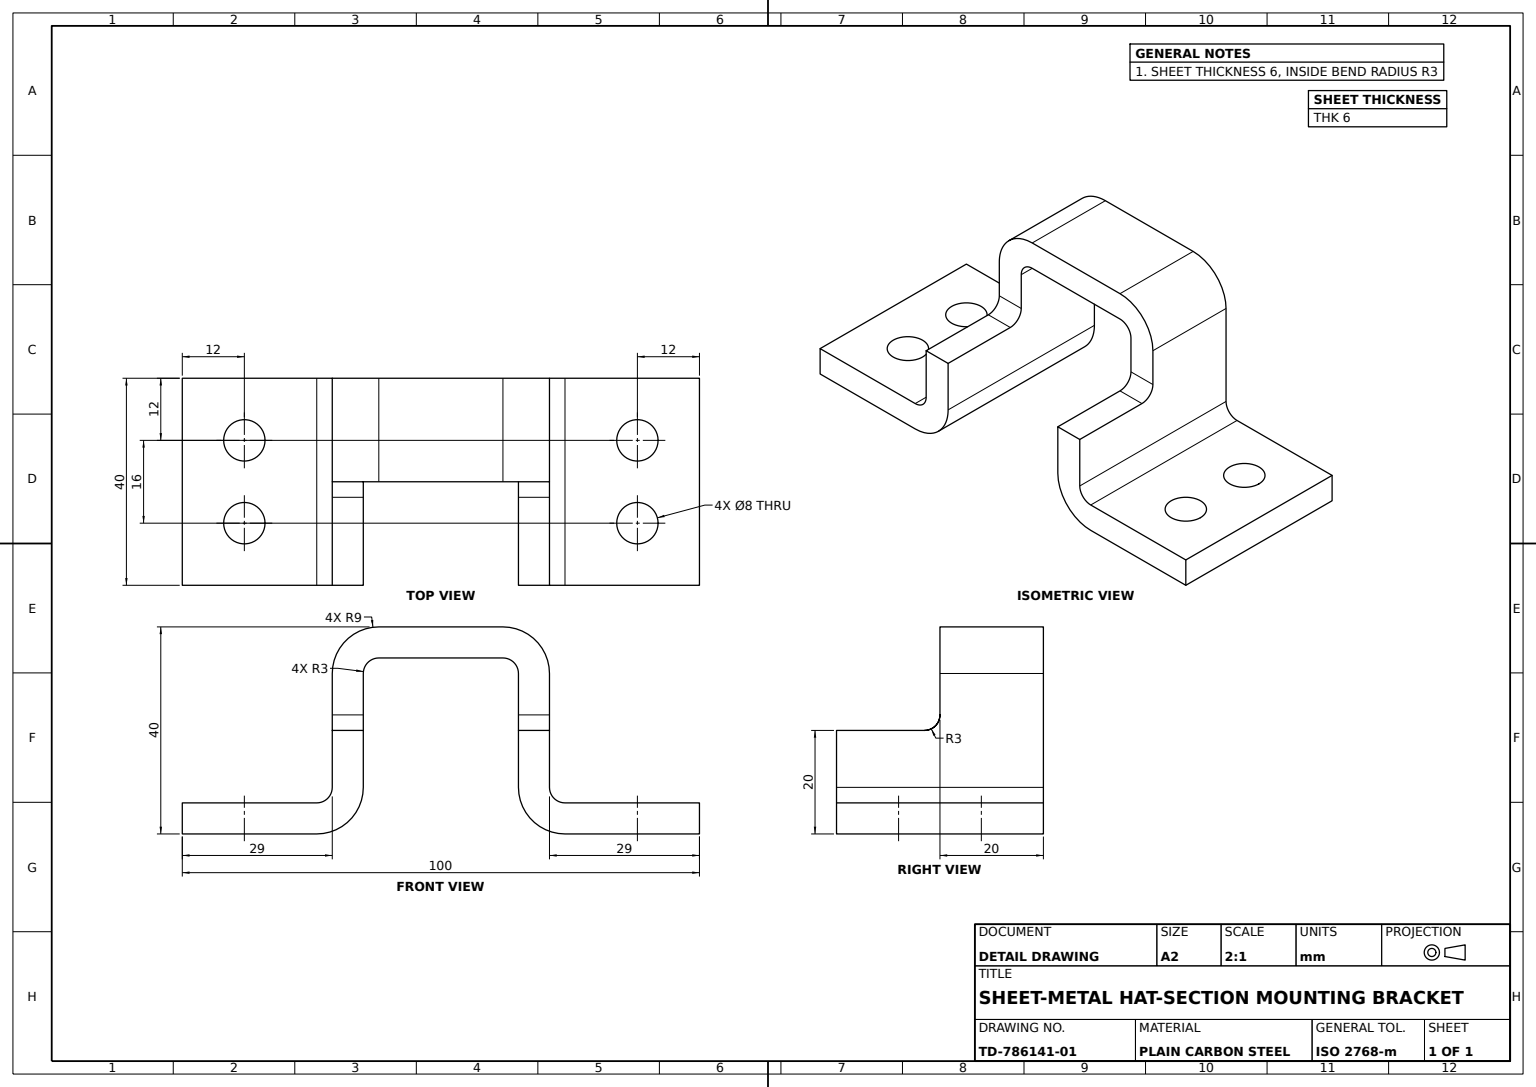
ISO-10303-21;
HEADER;
FILE_DESCRIPTION((''),'2;1');
FILE_NAME('','',(''),(''),'','','');
FILE_SCHEMA(('AUTOMOTIVE_DESIGN'));
ENDSEC;
DATA;
#1=APPLICATION_CONTEXT('');
#2=PRODUCT_CONTEXT('',#1,'mechanical');
#3=PRODUCT('','','',(#2));
#4=PRODUCT_DEFINITION_FORMATION('','',#3);
#5=PRODUCT_DEFINITION_CONTEXT('',#1,'design');
#6=PRODUCT_DEFINITION('','',#4,#5);
#7=PRODUCT_DEFINITION_SHAPE('','',#6);
#8=(LENGTH_UNIT()NAMED_UNIT(*)SI_UNIT(.MILLI.,.METRE.));
#9=(NAMED_UNIT(*)PLANE_ANGLE_UNIT()SI_UNIT($,.RADIAN.));
#10=(NAMED_UNIT(*)SI_UNIT($,.STERADIAN.)SOLID_ANGLE_UNIT());
#11=UNCERTAINTY_MEASURE_WITH_UNIT(LENGTH_MEASURE(1.E-05),#8,'distance_accuracy_value','');
#12=(GEOMETRIC_REPRESENTATION_CONTEXT(3)GLOBAL_UNCERTAINTY_ASSIGNED_CONTEXT((#11))GLOBAL_UNIT_ASSIGNED_CONTEXT((#8,#9,#10))REPRESENTATION_CONTEXT('',''));
#13=CARTESIAN_POINT('',(12.,6.,0.));
#14=VERTEX_POINT('',#13);
#15=CARTESIAN_POINT('',(12.,0.,0.));
#16=VERTEX_POINT('',#15);
#17=DIRECTION('',(0.,-1.,0.));
#18=VECTOR('',#17,1000.);
#19=LINE('',#13,#18);
#20=EDGE_CURVE('',#14,#16,#19,.T.);
#21=ORIENTED_EDGE('',*,*,#20,.F.);
#22=CARTESIAN_POINT('',(21.,-3.,0.));
#23=VERTEX_POINT('',#22);
#24=CARTESIAN_POINT('',(12.,-3.,0.));
#25=DIRECTION('',(0.,0.,-1.));
#26=DIRECTION('',(1.,0.,0.));
#27=AXIS2_PLACEMENT_3D('',#24,#25,#26);
#28=CIRCLE('',#27,9.);
#29=EDGE_CURVE('',#14,#23,#28,.T.);
#30=ORIENTED_EDGE('',*,*,#29,.T.);
#31=CARTESIAN_POINT('',(15.,-3.,0.));
#32=VERTEX_POINT('',#31);
#33=VECTOR('',#26,1000.);
#34=LINE('',#31,#33);
#35=EDGE_CURVE('',#32,#23,#34,.T.);
#36=ORIENTED_EDGE('',*,*,#35,.F.);
#37=CIRCLE('',#27,3.);
#38=EDGE_CURVE('',#16,#32,#37,.T.);
#39=ORIENTED_EDGE('',*,*,#38,.F.);
#40=EDGE_LOOP('',(#21,#30,#36,#39));
#41=FACE_OUTER_BOUND('',#40,.T.);
#42=DIRECTION('',(-1.,0.,0.));
#43=AXIS2_PLACEMENT_3D('',#31,#25,#42);
#44=PLANE('',#43);
#45=ADVANCED_FACE('',(#41),#44,.T.);
#46=CARTESIAN_POINT('',(-12.,6.,0.));
#47=VERTEX_POINT('',#46);
#48=CARTESIAN_POINT('',(15.,6.,0.));
#49=LINE('',#48,#33);
#50=EDGE_CURVE('',#47,#14,#49,.T.);
#51=ORIENTED_EDGE('',*,*,#50,.F.);
#52=CARTESIAN_POINT('',(-12.,6.,20.));
#53=VERTEX_POINT('',#52);
#54=CARTESIAN_POINT('',(-12.,6.,40.));
#55=VECTOR('',#25,1000.);
#56=LINE('',#54,#55);
#57=EDGE_CURVE('',#53,#47,#56,.T.);
#58=ORIENTED_EDGE('',*,*,#57,.F.);
#59=CARTESIAN_POINT('',(12.,6.,20.));
#60=VERTEX_POINT('',#59);
#61=CARTESIAN_POINT('',(-50.,6.,20.));
#62=LINE('',#61,#33);
#63=EDGE_CURVE('',#53,#60,#62,.T.);
#64=ORIENTED_EDGE('',*,*,#63,.T.);
#65=CARTESIAN_POINT('',(12.,6.,40.));
#66=LINE('',#65,#55);
#67=EDGE_CURVE('',#60,#14,#66,.T.);
#68=ORIENTED_EDGE('',*,*,#67,.T.);
#69=EDGE_LOOP('',(#51,#58,#64,#68));
#70=FACE_OUTER_BOUND('',#69,.T.);
#71=CARTESIAN_POINT('',(15.,6.,40.));
#72=DIRECTION('',(0.,1.,0.));
#73=DIRECTION('',(0.,0.,1.));
#74=AXIS2_PLACEMENT_3D('',#71,#72,#73);
#75=PLANE('',#74);
#76=ADVANCED_FACE('',(#70),#75,.T.);
#77=CARTESIAN_POINT('',(15.,-14.,40.));
#78=VERTEX_POINT('',#77);
#79=CARTESIAN_POINT('',(15.,-14.,23.));
#80=VERTEX_POINT('',#79);
#81=LINE('',#77,#55);
#82=EDGE_CURVE('',#78,#80,#81,.T.);
#83=ORIENTED_EDGE('',*,*,#82,.T.);
#84=CARTESIAN_POINT('',(15.,-11.,20.));
#85=VERTEX_POINT('',#84);
#86=CARTESIAN_POINT('',(15.,-11.,23.));
#87=AXIS2_PLACEMENT_3D('',#86,#26,#72);
#88=CIRCLE('',#87,3.);
#89=EDGE_CURVE('',#80,#85,#88,.T.);
#90=ORIENTED_EDGE('',*,*,#89,.T.);
#91=CARTESIAN_POINT('',(15.,-3.,20.));
#92=VERTEX_POINT('',#91);
#93=CARTESIAN_POINT('',(15.,0.,20.));
#94=VECTOR('',#72,1000.);
#95=LINE('',#93,#94);
#96=EDGE_CURVE('',#85,#92,#95,.T.);
#97=ORIENTED_EDGE('',*,*,#96,.T.);
#98=CARTESIAN_POINT('',(15.,-3.,40.));
#99=LINE('',#98,#55);
#100=EDGE_CURVE('',#92,#32,#99,.T.);
#101=ORIENTED_EDGE('',*,*,#100,.T.);
#102=CARTESIAN_POINT('',(15.,-25.,0.));
#103=VERTEX_POINT('',#102);
#104=CARTESIAN_POINT('',(15.,0.,0.));
#105=LINE('',#104,#18);
#106=EDGE_CURVE('',#32,#103,#105,.T.);
#107=ORIENTED_EDGE('',*,*,#106,.T.);
#108=CARTESIAN_POINT('',(15.,-25.,40.));
#109=VERTEX_POINT('',#108);
#110=LINE('',#108,#55);
#111=EDGE_CURVE('',#109,#103,#110,.T.);
#112=ORIENTED_EDGE('',*,*,#111,.F.);
#113=CARTESIAN_POINT('',(15.,0.,40.));
#114=LINE('',#113,#18);
#115=EDGE_CURVE('',#78,#109,#114,.T.);
#116=ORIENTED_EDGE('',*,*,#115,.F.);
#117=EDGE_LOOP('',(#83,#90,#97,#101,#107,#112,#116));
#118=FACE_OUTER_BOUND('',#117,.T.);
#119=AXIS2_PLACEMENT_3D('',#113,#26,#72);
#120=PLANE('',#119);
#121=ADVANCED_FACE('',(#118),#120,.F.);
#122=CARTESIAN_POINT('',(-50.,-34.,40.));
#123=VERTEX_POINT('',#122);
#124=CARTESIAN_POINT('',(-24.,-34.,40.));
#125=VERTEX_POINT('',#124);
#126=CARTESIAN_POINT('',(-15.,-34.,40.));
#127=LINE('',#126,#33);
#128=EDGE_CURVE('',#123,#125,#127,.T.);
#129=ORIENTED_EDGE('',*,*,#128,.T.);
#130=CARTESIAN_POINT('',(-24.,-28.,40.));
#131=VERTEX_POINT('',#130);
#132=LINE('',#124,#94);
#133=EDGE_CURVE('',#125,#131,#132,.T.);
#134=ORIENTED_EDGE('',*,*,#133,.T.);
#135=CARTESIAN_POINT('',(-50.,-28.,40.));
#136=VERTEX_POINT('',#135);
#137=CARTESIAN_POINT('',(-15.,-28.,40.));
#138=LINE('',#137,#33);
#139=EDGE_CURVE('',#136,#131,#138,.T.);
#140=ORIENTED_EDGE('',*,*,#139,.F.);
#141=LINE('',#122,#94);
#142=EDGE_CURVE('',#123,#136,#141,.T.);
#143=ORIENTED_EDGE('',*,*,#142,.F.);
#144=EDGE_LOOP('',(#129,#134,#140,#143));
#145=FACE_OUTER_BOUND('',#144,.T.);
#146=CARTESIAN_POINT('',(-21.,-25.,40.));
#147=AXIS2_PLACEMENT_3D('',#146,#73,#26);
#148=PLANE('',#147);
#149=ADVANCED_FACE('',(#145),#148,.T.);
#150=VERTEX_POINT('',#146);
#151=CARTESIAN_POINT('',(-24.,-25.,40.));
#152=AXIS2_PLACEMENT_3D('',#151,#73,#26);
#153=CIRCLE('',#152,3.);
#154=EDGE_CURVE('',#131,#150,#153,.T.);
#155=ORIENTED_EDGE('',*,*,#154,.T.);
#156=CARTESIAN_POINT('',(-21.,-25.,0.));
#157=VERTEX_POINT('',#156);
#158=LINE('',#146,#55);
#159=EDGE_CURVE('',#150,#157,#158,.T.);
#160=ORIENTED_EDGE('',*,*,#159,.T.);
#161=CARTESIAN_POINT('',(-24.,-28.,0.));
#162=VERTEX_POINT('',#161);
#163=CARTESIAN_POINT('',(-24.,-25.,0.));
#164=AXIS2_PLACEMENT_3D('',#163,#73,#26);
#165=CIRCLE('',#164,3.);
#166=EDGE_CURVE('',#162,#157,#165,.T.);
#167=ORIENTED_EDGE('',*,*,#166,.F.);
#168=LINE('',#130,#55);
#169=EDGE_CURVE('',#131,#162,#168,.T.);
#170=ORIENTED_EDGE('',*,*,#169,.F.);
#171=EDGE_LOOP('',(#155,#160,#167,#170));
#172=FACE_OUTER_BOUND('',#171,.T.);
#173=AXIS2_PLACEMENT_3D('',#151,#25,#42);
#174=CYLINDRICAL_SURFACE('',#173,3.);
#175=ADVANCED_FACE('',(#172),#174,.F.);
#176=CARTESIAN_POINT('',(-15.,-25.,40.));
#177=VERTEX_POINT('',#176);
#178=CARTESIAN_POINT('',(-15.,-25.,0.));
#179=VERTEX_POINT('',#178);
#180=LINE('',#176,#55);
#181=EDGE_CURVE('',#177,#179,#180,.T.);
#182=ORIENTED_EDGE('',*,*,#181,.F.);
#183=AXIS2_PLACEMENT_3D('',#151,#73,#42);
#184=CIRCLE('',#183,9.);
#185=EDGE_CURVE('',#125,#177,#184,.T.);
#186=ORIENTED_EDGE('',*,*,#185,.F.);
#187=CARTESIAN_POINT('',(-24.,-34.,0.));
#188=VERTEX_POINT('',#187);
#189=LINE('',#124,#55);
#190=EDGE_CURVE('',#125,#188,#189,.T.);
#191=ORIENTED_EDGE('',*,*,#190,.T.);
#192=AXIS2_PLACEMENT_3D('',#163,#73,#42);
#193=CIRCLE('',#192,9.);
#194=EDGE_CURVE('',#188,#179,#193,.T.);
#195=ORIENTED_EDGE('',*,*,#194,.T.);
#196=EDGE_LOOP('',(#182,#186,#191,#195));
#197=FACE_OUTER_BOUND('',#196,.T.);
#198=CYLINDRICAL_SURFACE('',#173,9.);
#199=ADVANCED_FACE('',(#197),#198,.T.);
#200=CARTESIAN_POINT('',(42.,-34.,12.));
#201=VERTEX_POINT('',#200);
#202=CARTESIAN_POINT('',(34.,-34.,12.));
#203=VERTEX_POINT('',#202);
#204=CARTESIAN_POINT('',(38.,-34.,12.));
#205=AXIS2_PLACEMENT_3D('',#204,#72,#42);
#206=CIRCLE('',#205,4.);
#207=EDGE_CURVE('',#201,#203,#206,.T.);
#208=ORIENTED_EDGE('',*,*,#207,.F.);
#209=CARTESIAN_POINT('',(42.,-28.,12.));
#210=VERTEX_POINT('',#209);
#211=LINE('',#200,#94);
#212=EDGE_CURVE('',#201,#210,#211,.T.);
#213=ORIENTED_EDGE('',*,*,#212,.T.);
#214=CARTESIAN_POINT('',(34.,-28.,12.));
#215=VERTEX_POINT('',#214);
#216=CARTESIAN_POINT('',(38.,-28.,12.));
#217=AXIS2_PLACEMENT_3D('',#216,#72,#42);
#218=CIRCLE('',#217,4.);
#219=EDGE_CURVE('',#210,#215,#218,.T.);
#220=ORIENTED_EDGE('',*,*,#219,.T.);
#221=LINE('',#202,#94);
#222=EDGE_CURVE('',#203,#215,#221,.T.);
#223=ORIENTED_EDGE('',*,*,#222,.F.);
#224=EDGE_LOOP('',(#208,#213,#220,#223));
#225=FACE_OUTER_BOUND('',#224,.T.);
#226=CYLINDRICAL_SURFACE('',#205,4.);
#227=ADVANCED_FACE('',(#225),#226,.F.);
#228=CARTESIAN_POINT('',(24.,-28.,40.));
#229=VERTEX_POINT('',#228);
#230=CARTESIAN_POINT('',(24.,-28.,0.));
#231=VERTEX_POINT('',#230);
#232=LINE('',#228,#55);
#233=EDGE_CURVE('',#229,#231,#232,.T.);
#234=ORIENTED_EDGE('',*,*,#233,.T.);
#235=CARTESIAN_POINT('',(21.,-25.,0.));
#236=VERTEX_POINT('',#235);
#237=CARTESIAN_POINT('',(24.,-25.,0.));
#238=AXIS2_PLACEMENT_3D('',#237,#73,#26);
#239=CIRCLE('',#238,3.);
#240=EDGE_CURVE('',#236,#231,#239,.T.);
#241=ORIENTED_EDGE('',*,*,#240,.F.);
#242=CARTESIAN_POINT('',(21.,-25.,40.));
#243=VERTEX_POINT('',#242);
#244=LINE('',#242,#55);
#245=EDGE_CURVE('',#243,#236,#244,.T.);
#246=ORIENTED_EDGE('',*,*,#245,.F.);
#247=CARTESIAN_POINT('',(24.,-25.,40.));
#248=AXIS2_PLACEMENT_3D('',#247,#73,#26);
#249=CIRCLE('',#248,3.);
#250=EDGE_CURVE('',#243,#229,#249,.T.);
#251=ORIENTED_EDGE('',*,*,#250,.T.);
#252=EDGE_LOOP('',(#234,#241,#246,#251));
#253=FACE_OUTER_BOUND('',#252,.T.);
#254=AXIS2_PLACEMENT_3D('',#247,#25,#42);
#255=CYLINDRICAL_SURFACE('',#254,3.);
#256=ADVANCED_FACE('',(#253),#255,.F.);
#257=CARTESIAN_POINT('',(-12.,0.,0.));
#258=VERTEX_POINT('',#257);
#259=LINE('',#257,#94);
#260=EDGE_CURVE('',#258,#47,#259,.T.);
#261=ORIENTED_EDGE('',*,*,#260,.T.);
#262=ORIENTED_EDGE('',*,*,#50,.T.);
#263=ORIENTED_EDGE('',*,*,#20,.T.);
#264=LINE('',#104,#33);
#265=EDGE_CURVE('',#258,#16,#264,.T.);
#266=ORIENTED_EDGE('',*,*,#265,.F.);
#267=EDGE_LOOP('',(#261,#262,#263,#266));
#268=FACE_OUTER_BOUND('',#267,.T.);
#269=CARTESIAN_POINT('',(-21.,-3.,0.));
#270=AXIS2_PLACEMENT_3D('',#269,#25,#42);
#271=PLANE('',#270);
#272=ADVANCED_FACE('',(#268),#271,.T.);
#273=LINE('',#161,#18);
#274=EDGE_CURVE('',#162,#188,#273,.T.);
#275=ORIENTED_EDGE('',*,*,#274,.T.);
#276=CARTESIAN_POINT('',(-50.,-34.,0.));
#277=VERTEX_POINT('',#276);
#278=CARTESIAN_POINT('',(-15.,-34.,0.));
#279=LINE('',#278,#33);
#280=EDGE_CURVE('',#277,#188,#279,.T.);
#281=ORIENTED_EDGE('',*,*,#280,.F.);
#282=CARTESIAN_POINT('',(-50.,-28.,0.));
#283=VERTEX_POINT('',#282);
#284=LINE('',#276,#94);
#285=EDGE_CURVE('',#277,#283,#284,.T.);
#286=ORIENTED_EDGE('',*,*,#285,.T.);
#287=CARTESIAN_POINT('',(-15.,-28.,0.));
#288=LINE('',#287,#33);
#289=EDGE_CURVE('',#283,#162,#288,.T.);
#290=ORIENTED_EDGE('',*,*,#289,.T.);
#291=EDGE_LOOP('',(#275,#281,#286,#290));
#292=FACE_OUTER_BOUND('',#291,.T.);
#293=PLANE('',#238);
#294=ADVANCED_FACE('',(#292),#293,.F.);
#295=ORIENTED_EDGE('',*,*,#194,.F.);
#296=ORIENTED_EDGE('',*,*,#274,.F.);
#297=ORIENTED_EDGE('',*,*,#166,.T.);
#298=VECTOR('',#42,1000.);
#299=LINE('',#178,#298);
#300=EDGE_CURVE('',#179,#157,#299,.T.);
#301=ORIENTED_EDGE('',*,*,#300,.F.);
#302=EDGE_LOOP('',(#295,#296,#297,#301));
#303=FACE_OUTER_BOUND('',#302,.T.);
#304=AXIS2_PLACEMENT_3D('',#178,#25,#42);
#305=PLANE('',#304);
#306=ADVANCED_FACE('',(#303),#305,.T.);
#307=LINE('',#146,#33);
#308=EDGE_CURVE('',#150,#177,#307,.T.);
#309=ORIENTED_EDGE('',*,*,#308,.F.);
#310=ORIENTED_EDGE('',*,*,#154,.F.);
#311=ORIENTED_EDGE('',*,*,#133,.F.);
#312=ORIENTED_EDGE('',*,*,#185,.T.);
#313=EDGE_LOOP('',(#309,#310,#311,#312));
#314=FACE_OUTER_BOUND('',#313,.T.);
#315=AXIS2_PLACEMENT_3D('',#124,#73,#26);
#316=PLANE('',#315);
#317=ADVANCED_FACE('',(#314),#316,.T.);
#318=CARTESIAN_POINT('',(21.,-3.,20.));
#319=VERTEX_POINT('',#318);
#320=CARTESIAN_POINT('',(12.,-3.,20.));
#321=AXIS2_PLACEMENT_3D('',#320,#73,#72);
#322=CIRCLE('',#321,9.);
#323=EDGE_CURVE('',#319,#60,#322,.T.);
#324=ORIENTED_EDGE('',*,*,#323,.F.);
#325=CARTESIAN_POINT('',(21.,-3.,40.));
#326=LINE('',#325,#55);
#327=EDGE_CURVE('',#319,#23,#326,.T.);
#328=ORIENTED_EDGE('',*,*,#327,.T.);
#329=ORIENTED_EDGE('',*,*,#29,.F.);
#330=ORIENTED_EDGE('',*,*,#67,.F.);
#331=EDGE_LOOP('',(#324,#328,#329,#330));
#332=FACE_OUTER_BOUND('',#331,.T.);
#333=CARTESIAN_POINT('',(12.,-3.,40.));
#334=AXIS2_PLACEMENT_3D('',#333,#25,#42);
#335=CYLINDRICAL_SURFACE('',#334,9.);
#336=ADVANCED_FACE('',(#332),#335,.T.);
#337=CARTESIAN_POINT('',(-12.,0.,20.));
#338=VERTEX_POINT('',#337);
#339=CARTESIAN_POINT('',(-15.,-3.,20.));
#340=VERTEX_POINT('',#339);
#341=CARTESIAN_POINT('',(-12.,-3.,20.));
#342=AXIS2_PLACEMENT_3D('',#341,#73,#72);
#343=CIRCLE('',#342,3.);
#344=EDGE_CURVE('',#338,#340,#343,.T.);
#345=ORIENTED_EDGE('',*,*,#344,.T.);
#346=CARTESIAN_POINT('',(-15.,-3.,0.));
#347=VERTEX_POINT('',#346);
#348=CARTESIAN_POINT('',(-15.,-3.,40.));
#349=LINE('',#348,#55);
#350=EDGE_CURVE('',#340,#347,#349,.T.);
#351=ORIENTED_EDGE('',*,*,#350,.T.);
#352=CARTESIAN_POINT('',(-12.,-3.,0.));
#353=AXIS2_PLACEMENT_3D('',#352,#25,#26);
#354=CIRCLE('',#353,3.);
#355=EDGE_CURVE('',#347,#258,#354,.T.);
#356=ORIENTED_EDGE('',*,*,#355,.T.);
#357=CARTESIAN_POINT('',(-12.,0.,40.));
#358=LINE('',#357,#55);
#359=EDGE_CURVE('',#338,#258,#358,.T.);
#360=ORIENTED_EDGE('',*,*,#359,.F.);
#361=EDGE_LOOP('',(#345,#351,#356,#360));
#362=FACE_OUTER_BOUND('',#361,.T.);
#363=CARTESIAN_POINT('',(-12.,-3.,40.));
#364=AXIS2_PLACEMENT_3D('',#363,#25,#42);
#365=CYLINDRICAL_SURFACE('',#364,3.);
#366=ADVANCED_FACE('',(#362),#365,.F.);
#367=LINE('',#135,#55);
#368=EDGE_CURVE('',#136,#283,#367,.T.);
#369=ORIENTED_EDGE('',*,*,#368,.T.);
#370=ORIENTED_EDGE('',*,*,#285,.F.);
#371=LINE('',#122,#55);
#372=EDGE_CURVE('',#123,#277,#371,.T.);
#373=ORIENTED_EDGE('',*,*,#372,.F.);
#374=ORIENTED_EDGE('',*,*,#142,.T.);
#375=EDGE_LOOP('',(#369,#370,#373,#374));
#376=FACE_OUTER_BOUND('',#375,.T.);
#377=AXIS2_PLACEMENT_3D('',#122,#42,#73);
#378=PLANE('',#377);
#379=ADVANCED_FACE('',(#376),#378,.T.);
#380=CARTESIAN_POINT('',(-34.,-28.,12.));
#381=VERTEX_POINT('',#380);
#382=CARTESIAN_POINT('',(-42.,-28.,12.));
#383=VERTEX_POINT('',#382);
#384=CARTESIAN_POINT('',(-38.,-28.,12.));
#385=AXIS2_PLACEMENT_3D('',#384,#72,#42);
#386=CIRCLE('',#385,4.);
#387=EDGE_CURVE('',#381,#383,#386,.T.);
#388=ORIENTED_EDGE('',*,*,#387,.T.);
#389=CARTESIAN_POINT('',(-42.,-34.,12.));
#390=VERTEX_POINT('',#389);
#391=LINE('',#389,#94);
#392=EDGE_CURVE('',#390,#383,#391,.T.);
#393=ORIENTED_EDGE('',*,*,#392,.F.);
#394=CARTESIAN_POINT('',(-34.,-34.,12.));
#395=VERTEX_POINT('',#394);
#396=CARTESIAN_POINT('',(-38.,-34.,12.));
#397=AXIS2_PLACEMENT_3D('',#396,#72,#42);
#398=CIRCLE('',#397,4.);
#399=EDGE_CURVE('',#395,#390,#398,.T.);
#400=ORIENTED_EDGE('',*,*,#399,.F.);
#401=LINE('',#394,#94);
#402=EDGE_CURVE('',#395,#381,#401,.T.);
#403=ORIENTED_EDGE('',*,*,#402,.T.);
#404=EDGE_LOOP('',(#388,#393,#400,#403));
#405=FACE_OUTER_BOUND('',#404,.T.);
#406=CYLINDRICAL_SURFACE('',#397,4.);
#407=ADVANCED_FACE('',(#405),#406,.F.);
#408=CARTESIAN_POINT('',(-34.,-34.,28.));
#409=VERTEX_POINT('',#408);
#410=CARTESIAN_POINT('',(-34.,-28.,28.));
#411=VERTEX_POINT('',#410);
#412=LINE('',#408,#94);
#413=EDGE_CURVE('',#409,#411,#412,.T.);
#414=ORIENTED_EDGE('',*,*,#413,.T.);
#415=CARTESIAN_POINT('',(-42.,-28.,28.));
#416=VERTEX_POINT('',#415);
#417=CARTESIAN_POINT('',(-38.,-28.,28.));
#418=AXIS2_PLACEMENT_3D('',#417,#72,#42);
#419=CIRCLE('',#418,4.);
#420=EDGE_CURVE('',#411,#416,#419,.T.);
#421=ORIENTED_EDGE('',*,*,#420,.T.);
#422=CARTESIAN_POINT('',(-42.,-34.,28.));
#423=VERTEX_POINT('',#422);
#424=LINE('',#422,#94);
#425=EDGE_CURVE('',#423,#416,#424,.T.);
#426=ORIENTED_EDGE('',*,*,#425,.F.);
#427=CARTESIAN_POINT('',(-38.,-34.,28.));
#428=AXIS2_PLACEMENT_3D('',#427,#72,#42);
#429=CIRCLE('',#428,4.);
#430=EDGE_CURVE('',#409,#423,#429,.T.);
#431=ORIENTED_EDGE('',*,*,#430,.F.);
#432=EDGE_LOOP('',(#414,#421,#426,#431));
#433=FACE_OUTER_BOUND('',#432,.T.);
#434=CYLINDRICAL_SURFACE('',#428,4.);
#435=ADVANCED_FACE('',(#433),#434,.F.);
#436=ORIENTED_EDGE('',*,*,#327,.F.);
#437=CARTESIAN_POINT('',(21.,-11.,20.));
#438=VERTEX_POINT('',#437);
#439=CARTESIAN_POINT('',(21.,0.,20.));
#440=LINE('',#439,#94);
#441=EDGE_CURVE('',#438,#319,#440,.T.);
#442=ORIENTED_EDGE('',*,*,#441,.F.);
#443=CARTESIAN_POINT('',(21.,-14.,23.));
#444=VERTEX_POINT('',#443);
#445=CARTESIAN_POINT('',(21.,-11.,23.));
#446=AXIS2_PLACEMENT_3D('',#445,#42,#72);
#447=CIRCLE('',#446,3.);
#448=EDGE_CURVE('',#438,#444,#447,.T.);
#449=ORIENTED_EDGE('',*,*,#448,.T.);
#450=CARTESIAN_POINT('',(21.,-14.,40.));
#451=VERTEX_POINT('',#450);
#452=LINE('',#450,#55);
#453=EDGE_CURVE('',#451,#444,#452,.T.);
#454=ORIENTED_EDGE('',*,*,#453,.F.);
#455=CARTESIAN_POINT('',(21.,0.,40.));
#456=LINE('',#455,#18);
#457=EDGE_CURVE('',#451,#243,#456,.T.);
#458=ORIENTED_EDGE('',*,*,#457,.T.);
#459=ORIENTED_EDGE('',*,*,#245,.T.);
#460=CARTESIAN_POINT('',(21.,0.,0.));
#461=LINE('',#460,#18);
#462=EDGE_CURVE('',#23,#236,#461,.T.);
#463=ORIENTED_EDGE('',*,*,#462,.F.);
#464=EDGE_LOOP('',(#436,#442,#449,#454,#458,#459,#463));
#465=FACE_OUTER_BOUND('',#464,.T.);
#466=AXIS2_PLACEMENT_3D('',#455,#26,#72);
#467=PLANE('',#466);
#468=ADVANCED_FACE('',(#465),#467,.T.);
#469=ORIENTED_EDGE('',*,*,#359,.T.);
#470=ORIENTED_EDGE('',*,*,#265,.T.);
#471=CARTESIAN_POINT('',(12.,0.,20.));
#472=VERTEX_POINT('',#471);
#473=CARTESIAN_POINT('',(12.,0.,40.));
#474=LINE('',#473,#55);
#475=EDGE_CURVE('',#472,#16,#474,.T.);
#476=ORIENTED_EDGE('',*,*,#475,.F.);
#477=LINE('',#93,#298);
#478=EDGE_CURVE('',#472,#338,#477,.T.);
#479=ORIENTED_EDGE('',*,*,#478,.T.);
#480=EDGE_LOOP('',(#469,#470,#476,#479));
#481=FACE_OUTER_BOUND('',#480,.T.);
#482=AXIS2_PLACEMENT_3D('',#113,#72,#73);
#483=PLANE('',#482);
#484=ADVANCED_FACE('',(#481),#483,.F.);
#485=CARTESIAN_POINT('',(24.,-34.,0.));
#486=VERTEX_POINT('',#485);
#487=LINE('',#485,#94);
#488=EDGE_CURVE('',#486,#231,#487,.T.);
#489=ORIENTED_EDGE('',*,*,#488,.F.);
#490=AXIS2_PLACEMENT_3D('',#237,#73,#42);
#491=CIRCLE('',#490,9.);
#492=EDGE_CURVE('',#103,#486,#491,.T.);
#493=ORIENTED_EDGE('',*,*,#492,.F.);
#494=LINE('',#235,#298);
#495=EDGE_CURVE('',#236,#103,#494,.T.);
#496=ORIENTED_EDGE('',*,*,#495,.F.);
#497=ORIENTED_EDGE('',*,*,#240,.T.);
#498=EDGE_LOOP('',(#489,#493,#496,#497));
#499=FACE_OUTER_BOUND('',#498,.T.);
#500=AXIS2_PLACEMENT_3D('',#485,#25,#42);
#501=PLANE('',#500);
#502=ADVANCED_FACE('',(#499),#501,.T.);
#503=EDGE_CURVE('',#423,#409,#429,.T.);
#504=ORIENTED_EDGE('',*,*,#503,.F.);
#505=ORIENTED_EDGE('',*,*,#425,.T.);
#506=EDGE_CURVE('',#416,#411,#419,.T.);
#507=ORIENTED_EDGE('',*,*,#506,.T.);
#508=ORIENTED_EDGE('',*,*,#413,.F.);
#509=EDGE_LOOP('',(#504,#505,#507,#508));
#510=FACE_OUTER_BOUND('',#509,.T.);
#511=ADVANCED_FACE('',(#510),#434,.F.);
#512=VERTEX_POINT('',#269);
#513=LINE('',#269,#33);
#514=EDGE_CURVE('',#512,#347,#513,.T.);
#515=ORIENTED_EDGE('',*,*,#514,.F.);
#516=CIRCLE('',#353,9.);
#517=EDGE_CURVE('',#512,#47,#516,.T.);
#518=ORIENTED_EDGE('',*,*,#517,.T.);
#519=ORIENTED_EDGE('',*,*,#260,.F.);
#520=ORIENTED_EDGE('',*,*,#355,.F.);
#521=EDGE_LOOP('',(#515,#518,#519,#520));
#522=FACE_OUTER_BOUND('',#521,.T.);
#523=AXIS2_PLACEMENT_3D('',#257,#25,#42);
#524=PLANE('',#523);
#525=ADVANCED_FACE('',(#522),#524,.T.);
#526=CARTESIAN_POINT('',(-21.,0.,0.));
#527=LINE('',#526,#94);
#528=EDGE_CURVE('',#157,#512,#527,.T.);
#529=ORIENTED_EDGE('',*,*,#528,.T.);
#530=ORIENTED_EDGE('',*,*,#514,.T.);
#531=CARTESIAN_POINT('',(-15.,0.,0.));
#532=LINE('',#531,#94);
#533=EDGE_CURVE('',#179,#347,#532,.T.);
#534=ORIENTED_EDGE('',*,*,#533,.F.);
#535=ORIENTED_EDGE('',*,*,#300,.T.);
#536=EDGE_LOOP('',(#529,#530,#534,#535));
#537=FACE_OUTER_BOUND('',#536,.T.);
#538=AXIS2_PLACEMENT_3D('',#161,#25,#42);
#539=PLANE('',#538);
#540=ADVANCED_FACE('',(#537),#539,.T.);
#541=ORIENTED_EDGE('',*,*,#475,.T.);
#542=ORIENTED_EDGE('',*,*,#38,.T.);
#543=ORIENTED_EDGE('',*,*,#100,.F.);
#544=CIRCLE('',#321,3.);
#545=EDGE_CURVE('',#92,#472,#544,.T.);
#546=ORIENTED_EDGE('',*,*,#545,.T.);
#547=EDGE_LOOP('',(#541,#542,#543,#546));
#548=FACE_OUTER_BOUND('',#547,.T.);
#549=CYLINDRICAL_SURFACE('',#334,3.);
#550=ADVANCED_FACE('',(#548),#549,.F.);
#551=CARTESIAN_POINT('',(-21.,-14.,23.));
#552=VERTEX_POINT('',#551);
#553=CARTESIAN_POINT('',(-21.,-11.,20.));
#554=VERTEX_POINT('',#553);
#555=CARTESIAN_POINT('',(-21.,-11.,23.));
#556=AXIS2_PLACEMENT_3D('',#555,#26,#17);
#557=CIRCLE('',#556,3.);
#558=EDGE_CURVE('',#552,#554,#557,.T.);
#559=ORIENTED_EDGE('',*,*,#558,.F.);
#560=CARTESIAN_POINT('',(-15.,-14.,23.));
#561=VERTEX_POINT('',#560);
#562=LINE('',#551,#298);
#563=EDGE_CURVE('',#561,#552,#562,.T.);
#564=ORIENTED_EDGE('',*,*,#563,.F.);
#565=CARTESIAN_POINT('',(-15.,-11.,20.));
#566=VERTEX_POINT('',#565);
#567=CARTESIAN_POINT('',(-15.,-11.,23.));
#568=AXIS2_PLACEMENT_3D('',#567,#42,#17);
#569=CIRCLE('',#568,3.);
#570=EDGE_CURVE('',#566,#561,#569,.T.);
#571=ORIENTED_EDGE('',*,*,#570,.F.);
#572=LINE('',#565,#33);
#573=EDGE_CURVE('',#554,#566,#572,.T.);
#574=ORIENTED_EDGE('',*,*,#573,.F.);
#575=EDGE_LOOP('',(#559,#564,#571,#574));
#576=FACE_OUTER_BOUND('',#575,.T.);
#577=CARTESIAN_POINT('',(-50.,-11.,23.));
#578=AXIS2_PLACEMENT_3D('',#577,#42,#73);
#579=CYLINDRICAL_SURFACE('',#578,3.);
#580=ADVANCED_FACE('',(#576),#579,.F.);
#581=CARTESIAN_POINT('',(50.,-28.,40.));
#582=VERTEX_POINT('',#581);
#583=CARTESIAN_POINT('',(50.,-28.,0.));
#584=VERTEX_POINT('',#583);
#585=LINE('',#581,#55);
#586=EDGE_CURVE('',#582,#584,#585,.T.);
#587=ORIENTED_EDGE('',*,*,#586,.T.);
#588=CARTESIAN_POINT('',(15.,-28.,0.));
#589=LINE('',#588,#33);
#590=EDGE_CURVE('',#231,#584,#589,.T.);
#591=ORIENTED_EDGE('',*,*,#590,.F.);
#592=ORIENTED_EDGE('',*,*,#233,.F.);
#593=CARTESIAN_POINT('',(15.,-28.,40.));
#594=LINE('',#593,#33);
#595=EDGE_CURVE('',#229,#582,#594,.T.);
#596=ORIENTED_EDGE('',*,*,#595,.T.);
#597=EDGE_LOOP('',(#587,#591,#592,#596));
#598=FACE_OUTER_BOUND('',#597,.T.);
#599=CARTESIAN_POINT('',(34.,-28.,28.));
#600=VERTEX_POINT('',#599);
#601=CARTESIAN_POINT('',(42.,-28.,28.));
#602=VERTEX_POINT('',#601);
#603=CARTESIAN_POINT('',(38.,-28.,28.));
#604=AXIS2_PLACEMENT_3D('',#603,#72,#42);
#605=CIRCLE('',#604,4.);
#606=EDGE_CURVE('',#600,#602,#605,.T.);
#607=ORIENTED_EDGE('',*,*,#606,.F.);
#608=EDGE_CURVE('',#602,#600,#605,.T.);
#609=ORIENTED_EDGE('',*,*,#608,.F.);
#610=EDGE_LOOP('',(#607,#609));
#611=FACE_BOUND('',#610,.T.);
#612=EDGE_CURVE('',#215,#210,#218,.T.);
#613=ORIENTED_EDGE('',*,*,#612,.F.);
#614=ORIENTED_EDGE('',*,*,#219,.F.);
#615=EDGE_LOOP('',(#613,#614));
#616=FACE_BOUND('',#615,.T.);
#617=AXIS2_PLACEMENT_3D('',#593,#72,#42);
#618=PLANE('',#617);
#619=ADVANCED_FACE('',(#598,#611,#616),#618,.T.);
#620=ORIENTED_EDGE('',*,*,#457,.F.);
#621=CARTESIAN_POINT('',(-50.,-14.,40.));
#622=LINE('',#621,#33);
#623=EDGE_CURVE('',#78,#451,#622,.T.);
#624=ORIENTED_EDGE('',*,*,#623,.F.);
#625=ORIENTED_EDGE('',*,*,#115,.T.);
#626=LINE('',#108,#33);
#627=EDGE_CURVE('',#109,#243,#626,.T.);
#628=ORIENTED_EDGE('',*,*,#627,.T.);
#629=EDGE_LOOP('',(#620,#624,#625,#628));
#630=FACE_OUTER_BOUND('',#629,.T.);
#631=AXIS2_PLACEMENT_3D('',#228,#73,#26);
#632=PLANE('',#631);
#633=ADVANCED_FACE('',(#630),#632,.T.);
#634=CARTESIAN_POINT('',(-21.,-14.,40.));
#635=VERTEX_POINT('',#634);
#636=VECTOR('',#73,1000.);
#637=LINE('',#634,#636);
#638=EDGE_CURVE('',#552,#635,#637,.T.);
#639=ORIENTED_EDGE('',*,*,#638,.T.);
#640=CARTESIAN_POINT('',(-15.,-14.,40.));
#641=VERTEX_POINT('',#640);
#642=EDGE_CURVE('',#635,#641,#622,.T.);
#643=ORIENTED_EDGE('',*,*,#642,.T.);
#644=LINE('',#640,#636);
#645=EDGE_CURVE('',#561,#641,#644,.T.);
#646=ORIENTED_EDGE('',*,*,#645,.F.);
#647=ORIENTED_EDGE('',*,*,#563,.T.);
#648=EDGE_LOOP('',(#639,#643,#646,#647));
#649=FACE_OUTER_BOUND('',#648,.T.);
#650=AXIS2_PLACEMENT_3D('',#621,#17,#25);
#651=PLANE('',#650);
#652=ADVANCED_FACE('',(#649),#651,.F.);
#653=LINE('',#52,#18);
#654=EDGE_CURVE('',#53,#338,#653,.T.);
#655=ORIENTED_EDGE('',*,*,#654,.T.);
#656=ORIENTED_EDGE('',*,*,#478,.F.);
#657=LINE('',#471,#94);
#658=EDGE_CURVE('',#472,#60,#657,.T.);
#659=ORIENTED_EDGE('',*,*,#658,.T.);
#660=ORIENTED_EDGE('',*,*,#63,.F.);
#661=EDGE_LOOP('',(#655,#656,#659,#660));
#662=FACE_OUTER_BOUND('',#661,.T.);
#663=AXIS2_PLACEMENT_3D('',#61,#25,#72);
#664=PLANE('',#663);
#665=ADVANCED_FACE('',(#662),#664,.F.);
#666=ORIENTED_EDGE('',*,*,#350,.F.);
#667=CARTESIAN_POINT('',(-15.,0.,20.));
#668=LINE('',#667,#18);
#669=EDGE_CURVE('',#340,#566,#668,.T.);
#670=ORIENTED_EDGE('',*,*,#669,.T.);
#671=ORIENTED_EDGE('',*,*,#570,.T.);
#672=ORIENTED_EDGE('',*,*,#645,.T.);
#673=CARTESIAN_POINT('',(-15.,0.,40.));
#674=LINE('',#673,#94);
#675=EDGE_CURVE('',#177,#641,#674,.T.);
#676=ORIENTED_EDGE('',*,*,#675,.F.);
#677=ORIENTED_EDGE('',*,*,#181,.T.);
#678=ORIENTED_EDGE('',*,*,#533,.T.);
#679=EDGE_LOOP('',(#666,#670,#671,#672,#676,#677,#678));
#680=FACE_OUTER_BOUND('',#679,.T.);
#681=AXIS2_PLACEMENT_3D('',#673,#42,#17);
#682=PLANE('',#681);
#683=ADVANCED_FACE('',(#680),#682,.F.);
#684=ORIENTED_EDGE('',*,*,#627,.F.);
#685=CARTESIAN_POINT('',(24.,-34.,40.));
#686=VERTEX_POINT('',#685);
#687=AXIS2_PLACEMENT_3D('',#247,#73,#42);
#688=CIRCLE('',#687,9.);
#689=EDGE_CURVE('',#109,#686,#688,.T.);
#690=ORIENTED_EDGE('',*,*,#689,.T.);
#691=LINE('',#228,#18);
#692=EDGE_CURVE('',#229,#686,#691,.T.);
#693=ORIENTED_EDGE('',*,*,#692,.F.);
#694=ORIENTED_EDGE('',*,*,#250,.F.);
#695=EDGE_LOOP('',(#684,#690,#693,#694));
#696=FACE_OUTER_BOUND('',#695,.T.);
#697=AXIS2_PLACEMENT_3D('',#108,#73,#26);
#698=PLANE('',#697);
#699=ADVANCED_FACE('',(#696),#698,.T.);
#700=ORIENTED_EDGE('',*,*,#35,.T.);
#701=ORIENTED_EDGE('',*,*,#462,.T.);
#702=ORIENTED_EDGE('',*,*,#495,.T.);
#703=ORIENTED_EDGE('',*,*,#106,.F.);
#704=EDGE_LOOP('',(#700,#701,#702,#703));
#705=FACE_OUTER_BOUND('',#704,.T.);
#706=AXIS2_PLACEMENT_3D('',#13,#25,#42);
#707=PLANE('',#706);
#708=ADVANCED_FACE('',(#705),#707,.T.);
#709=ORIENTED_EDGE('',*,*,#689,.F.);
#710=ORIENTED_EDGE('',*,*,#111,.T.);
#711=ORIENTED_EDGE('',*,*,#492,.T.);
#712=LINE('',#685,#55);
#713=EDGE_CURVE('',#686,#486,#712,.T.);
#714=ORIENTED_EDGE('',*,*,#713,.F.);
#715=EDGE_LOOP('',(#709,#710,#711,#714));
#716=FACE_OUTER_BOUND('',#715,.T.);
#717=CYLINDRICAL_SURFACE('',#254,9.);
#718=ADVANCED_FACE('',(#716),#717,.T.);
#719=ORIENTED_EDGE('',*,*,#528,.F.);
#720=ORIENTED_EDGE('',*,*,#159,.F.);
#721=CARTESIAN_POINT('',(-21.,0.,40.));
#722=LINE('',#721,#94);
#723=EDGE_CURVE('',#150,#635,#722,.T.);
#724=ORIENTED_EDGE('',*,*,#723,.T.);
#725=ORIENTED_EDGE('',*,*,#638,.F.);
#726=ORIENTED_EDGE('',*,*,#558,.T.);
#727=CARTESIAN_POINT('',(-21.,-3.,20.));
#728=VERTEX_POINT('',#727);
#729=CARTESIAN_POINT('',(-21.,0.,20.));
#730=LINE('',#729,#18);
#731=EDGE_CURVE('',#728,#554,#730,.T.);
#732=ORIENTED_EDGE('',*,*,#731,.F.);
#733=CARTESIAN_POINT('',(-21.,-3.,40.));
#734=LINE('',#733,#55);
#735=EDGE_CURVE('',#728,#512,#734,.T.);
#736=ORIENTED_EDGE('',*,*,#735,.T.);
#737=EDGE_LOOP('',(#719,#720,#724,#725,#726,#732,#736));
#738=FACE_OUTER_BOUND('',#737,.T.);
#739=AXIS2_PLACEMENT_3D('',#721,#42,#17);
#740=PLANE('',#739);
#741=ADVANCED_FACE('',(#738),#740,.T.);
#742=ORIENTED_EDGE('',*,*,#723,.F.);
#743=ORIENTED_EDGE('',*,*,#308,.T.);
#744=ORIENTED_EDGE('',*,*,#675,.T.);
#745=ORIENTED_EDGE('',*,*,#642,.F.);
#746=EDGE_LOOP('',(#742,#743,#744,#745));
#747=FACE_OUTER_BOUND('',#746,.T.);
#748=AXIS2_PLACEMENT_3D('',#54,#73,#26);
#749=PLANE('',#748);
#750=ADVANCED_FACE('',(#747),#749,.T.);
#751=CARTESIAN_POINT('',(50.,-34.,0.));
#752=VERTEX_POINT('',#751);
#753=LINE('',#583,#18);
#754=EDGE_CURVE('',#584,#752,#753,.T.);
#755=ORIENTED_EDGE('',*,*,#754,.F.);
#756=ORIENTED_EDGE('',*,*,#586,.F.);
#757=CARTESIAN_POINT('',(50.,-34.,40.));
#758=VERTEX_POINT('',#757);
#759=LINE('',#581,#18);
#760=EDGE_CURVE('',#582,#758,#759,.T.);
#761=ORIENTED_EDGE('',*,*,#760,.T.);
#762=LINE('',#757,#55);
#763=EDGE_CURVE('',#758,#752,#762,.T.);
#764=ORIENTED_EDGE('',*,*,#763,.T.);
#765=EDGE_LOOP('',(#755,#756,#761,#764));
#766=FACE_OUTER_BOUND('',#765,.T.);
#767=AXIS2_PLACEMENT_3D('',#581,#26,#25);
#768=PLANE('',#767);
#769=ADVANCED_FACE('',(#766),#768,.T.);
#770=ORIENTED_EDGE('',*,*,#82,.F.);
#771=ORIENTED_EDGE('',*,*,#623,.T.);
#772=ORIENTED_EDGE('',*,*,#453,.T.);
#773=LINE('',#79,#298);
#774=EDGE_CURVE('',#444,#80,#773,.T.);
#775=ORIENTED_EDGE('',*,*,#774,.T.);
#776=EDGE_LOOP('',(#770,#771,#772,#775));
#777=FACE_OUTER_BOUND('',#776,.T.);
#778=ADVANCED_FACE('',(#777),#651,.F.);
#779=ORIENTED_EDGE('',*,*,#344,.F.);
#780=ORIENTED_EDGE('',*,*,#654,.F.);
#781=CIRCLE('',#342,9.);
#782=EDGE_CURVE('',#53,#728,#781,.T.);
#783=ORIENTED_EDGE('',*,*,#782,.T.);
#784=LINE('',#339,#298);
#785=EDGE_CURVE('',#340,#728,#784,.T.);
#786=ORIENTED_EDGE('',*,*,#785,.F.);
#787=EDGE_LOOP('',(#779,#780,#783,#786));
#788=FACE_OUTER_BOUND('',#787,.T.);
#789=ADVANCED_FACE('',(#788),#664,.F.);
#790=ORIENTED_EDGE('',*,*,#368,.F.);
#791=ORIENTED_EDGE('',*,*,#139,.T.);
#792=ORIENTED_EDGE('',*,*,#169,.T.);
#793=ORIENTED_EDGE('',*,*,#289,.F.);
#794=EDGE_LOOP('',(#790,#791,#792,#793));
#795=FACE_OUTER_BOUND('',#794,.T.);
#796=ORIENTED_EDGE('',*,*,#387,.F.);
#797=EDGE_CURVE('',#383,#381,#386,.T.);
#798=ORIENTED_EDGE('',*,*,#797,.F.);
#799=EDGE_LOOP('',(#796,#798));
#800=FACE_BOUND('',#799,.T.);
#801=ORIENTED_EDGE('',*,*,#506,.F.);
#802=ORIENTED_EDGE('',*,*,#420,.F.);
#803=EDGE_LOOP('',(#801,#802));
#804=FACE_BOUND('',#803,.T.);
#805=AXIS2_PLACEMENT_3D('',#137,#72,#42);
#806=PLANE('',#805);
#807=ADVANCED_FACE('',(#795,#800,#804),#806,.T.);
#808=ORIENTED_EDGE('',*,*,#190,.F.);
#809=ORIENTED_EDGE('',*,*,#128,.F.);
#810=ORIENTED_EDGE('',*,*,#372,.T.);
#811=ORIENTED_EDGE('',*,*,#280,.T.);
#812=EDGE_LOOP('',(#808,#809,#810,#811));
#813=FACE_OUTER_BOUND('',#812,.T.);
#814=ORIENTED_EDGE('',*,*,#399,.T.);
#815=EDGE_CURVE('',#390,#395,#398,.T.);
#816=ORIENTED_EDGE('',*,*,#815,.T.);
#817=EDGE_LOOP('',(#814,#816));
#818=FACE_BOUND('',#817,.T.);
#819=ORIENTED_EDGE('',*,*,#503,.T.);
#820=ORIENTED_EDGE('',*,*,#430,.T.);
#821=EDGE_LOOP('',(#819,#820));
#822=FACE_BOUND('',#821,.T.);
#823=AXIS2_PLACEMENT_3D('',#126,#72,#42);
#824=PLANE('',#823);
#825=ADVANCED_FACE('',(#813,#818,#822),#824,.F.);
#826=ORIENTED_EDGE('',*,*,#760,.F.);
#827=ORIENTED_EDGE('',*,*,#595,.F.);
#828=ORIENTED_EDGE('',*,*,#692,.T.);
#829=CARTESIAN_POINT('',(15.,-34.,40.));
#830=LINE('',#829,#33);
#831=EDGE_CURVE('',#686,#758,#830,.T.);
#832=ORIENTED_EDGE('',*,*,#831,.T.);
#833=EDGE_LOOP('',(#826,#827,#828,#832));
#834=FACE_OUTER_BOUND('',#833,.T.);
#835=PLANE('',#248);
#836=ADVANCED_FACE('',(#834),#835,.T.);
#837=ORIENTED_EDGE('',*,*,#402,.F.);
#838=ORIENTED_EDGE('',*,*,#815,.F.);
#839=ORIENTED_EDGE('',*,*,#392,.T.);
#840=ORIENTED_EDGE('',*,*,#797,.T.);
#841=EDGE_LOOP('',(#837,#838,#839,#840));
#842=FACE_OUTER_BOUND('',#841,.T.);
#843=ADVANCED_FACE('',(#842),#406,.F.);
#844=CARTESIAN_POINT('',(42.,-34.,28.));
#845=VERTEX_POINT('',#844);
#846=LINE('',#844,#94);
#847=EDGE_CURVE('',#845,#602,#846,.T.);
#848=ORIENTED_EDGE('',*,*,#847,.T.);
#849=ORIENTED_EDGE('',*,*,#608,.T.);
#850=CARTESIAN_POINT('',(34.,-34.,28.));
#851=VERTEX_POINT('',#850);
#852=LINE('',#850,#94);
#853=EDGE_CURVE('',#851,#600,#852,.T.);
#854=ORIENTED_EDGE('',*,*,#853,.F.);
#855=CARTESIAN_POINT('',(38.,-34.,28.));
#856=AXIS2_PLACEMENT_3D('',#855,#72,#42);
#857=CIRCLE('',#856,4.);
#858=EDGE_CURVE('',#845,#851,#857,.T.);
#859=ORIENTED_EDGE('',*,*,#858,.F.);
#860=EDGE_LOOP('',(#848,#849,#854,#859));
#861=FACE_OUTER_BOUND('',#860,.T.);
#862=CYLINDRICAL_SURFACE('',#856,4.);
#863=ADVANCED_FACE('',(#861),#862,.F.);
#864=ORIENTED_EDGE('',*,*,#731,.T.);
#865=ORIENTED_EDGE('',*,*,#573,.T.);
#866=ORIENTED_EDGE('',*,*,#669,.F.);
#867=ORIENTED_EDGE('',*,*,#785,.T.);
#868=EDGE_LOOP('',(#864,#865,#866,#867));
#869=FACE_OUTER_BOUND('',#868,.T.);
#870=ADVANCED_FACE('',(#869),#664,.F.);
#871=ORIENTED_EDGE('',*,*,#754,.T.);
#872=CARTESIAN_POINT('',(15.,-34.,0.));
#873=LINE('',#872,#33);
#874=EDGE_CURVE('',#486,#752,#873,.T.);
#875=ORIENTED_EDGE('',*,*,#874,.F.);
#876=ORIENTED_EDGE('',*,*,#488,.T.);
#877=ORIENTED_EDGE('',*,*,#590,.T.);
#878=EDGE_LOOP('',(#871,#875,#876,#877));
#879=FACE_OUTER_BOUND('',#878,.T.);
#880=AXIS2_PLACEMENT_3D('',#235,#25,#42);
#881=PLANE('',#880);
#882=ADVANCED_FACE('',(#879),#881,.T.);
#883=LINE('',#318,#298);
#884=EDGE_CURVE('',#319,#92,#883,.T.);
#885=ORIENTED_EDGE('',*,*,#884,.F.);
#886=ORIENTED_EDGE('',*,*,#323,.T.);
#887=ORIENTED_EDGE('',*,*,#658,.F.);
#888=ORIENTED_EDGE('',*,*,#545,.F.);
#889=EDGE_LOOP('',(#885,#886,#887,#888));
#890=FACE_OUTER_BOUND('',#889,.T.);
#891=ADVANCED_FACE('',(#890),#664,.F.);
#892=ORIENTED_EDGE('',*,*,#606,.T.);
#893=ORIENTED_EDGE('',*,*,#847,.F.);
#894=EDGE_CURVE('',#851,#845,#857,.T.);
#895=ORIENTED_EDGE('',*,*,#894,.F.);
#896=ORIENTED_EDGE('',*,*,#853,.T.);
#897=EDGE_LOOP('',(#892,#893,#895,#896));
#898=FACE_OUTER_BOUND('',#897,.T.);
#899=ADVANCED_FACE('',(#898),#862,.F.);
#900=ORIENTED_EDGE('',*,*,#782,.F.);
#901=ORIENTED_EDGE('',*,*,#57,.T.);
#902=ORIENTED_EDGE('',*,*,#517,.F.);
#903=ORIENTED_EDGE('',*,*,#735,.F.);
#904=EDGE_LOOP('',(#900,#901,#902,#903));
#905=FACE_OUTER_BOUND('',#904,.T.);
#906=CYLINDRICAL_SURFACE('',#364,9.);
#907=ADVANCED_FACE('',(#905),#906,.T.);
#908=LINE('',#437,#33);
#909=EDGE_CURVE('',#85,#438,#908,.T.);
#910=ORIENTED_EDGE('',*,*,#909,.T.);
#911=ORIENTED_EDGE('',*,*,#441,.T.);
#912=ORIENTED_EDGE('',*,*,#884,.T.);
#913=ORIENTED_EDGE('',*,*,#96,.F.);
#914=EDGE_LOOP('',(#910,#911,#912,#913));
#915=FACE_OUTER_BOUND('',#914,.T.);
#916=ADVANCED_FACE('',(#915),#664,.F.);
#917=ORIENTED_EDGE('',*,*,#858,.T.);
#918=ORIENTED_EDGE('',*,*,#894,.T.);
#919=EDGE_LOOP('',(#917,#918));
#920=FACE_BOUND('',#919,.T.);
#921=ORIENTED_EDGE('',*,*,#874,.T.);
#922=ORIENTED_EDGE('',*,*,#763,.F.);
#923=ORIENTED_EDGE('',*,*,#831,.F.);
#924=ORIENTED_EDGE('',*,*,#713,.T.);
#925=EDGE_LOOP('',(#921,#922,#923,#924));
#926=FACE_OUTER_BOUND('',#925,.T.);
#927=EDGE_CURVE('',#203,#201,#206,.T.);
#928=ORIENTED_EDGE('',*,*,#927,.T.);
#929=ORIENTED_EDGE('',*,*,#207,.T.);
#930=EDGE_LOOP('',(#928,#929));
#931=FACE_BOUND('',#930,.T.);
#932=AXIS2_PLACEMENT_3D('',#829,#72,#42);
#933=PLANE('',#932);
#934=ADVANCED_FACE('',(#920,#926,#931),#933,.F.);
#935=ORIENTED_EDGE('',*,*,#89,.F.);
#936=ORIENTED_EDGE('',*,*,#774,.F.);
#937=ORIENTED_EDGE('',*,*,#448,.F.);
#938=ORIENTED_EDGE('',*,*,#909,.F.);
#939=EDGE_LOOP('',(#935,#936,#937,#938));
#940=FACE_OUTER_BOUND('',#939,.T.);
#941=ADVANCED_FACE('',(#940),#579,.F.);
#942=ORIENTED_EDGE('',*,*,#212,.F.);
#943=ORIENTED_EDGE('',*,*,#927,.F.);
#944=ORIENTED_EDGE('',*,*,#222,.T.);
#945=ORIENTED_EDGE('',*,*,#612,.T.);
#946=EDGE_LOOP('',(#942,#943,#944,#945));
#947=FACE_OUTER_BOUND('',#946,.T.);
#948=ADVANCED_FACE('',(#947),#226,.F.);
#949=CLOSED_SHELL('',(#45,#76,#121,#149,#175,#199,#227,#256,#272,#294,#306,#317,#336,#366,#379,#407,#435,#468,#484,#502,#511,#525,#540,#550,#580,#619,#633,#652,#665,#683,#699,#708,#718,#741,#750,#769,#778,#789,#807,#825,#836,#843,#863,#870,#882,#891,#899,#907,#916,#934,#941,#948));
#950=MANIFOLD_SOLID_BREP('',#949);
#951=ADVANCED_BREP_SHAPE_REPRESENTATION('',(#950),#12);
#952=SHAPE_DEFINITION_REPRESENTATION(#7,#951);
ENDSEC;
END-ISO-10303-21;
